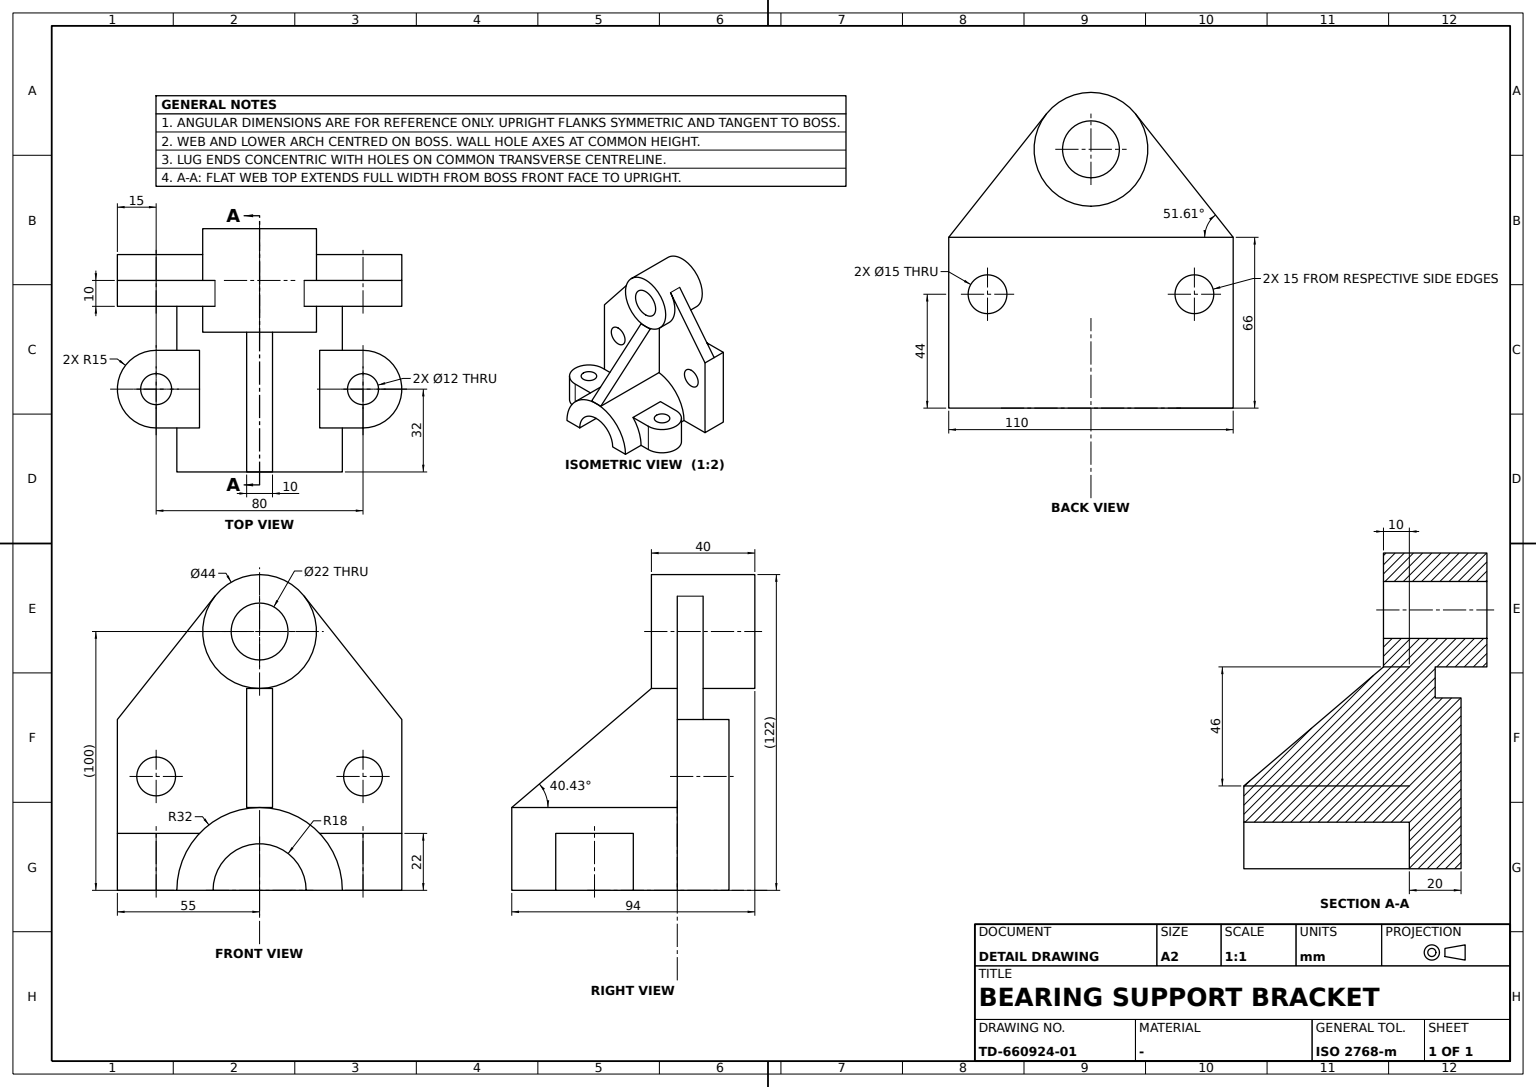
ISO-10303-21;
HEADER;
FILE_DESCRIPTION((''),'2;1');
FILE_NAME('','',(''),(''),'','','');
FILE_SCHEMA(('AUTOMOTIVE_DESIGN'));
ENDSEC;
DATA;
#1=APPLICATION_CONTEXT('');
#2=PRODUCT_CONTEXT('',#1,'mechanical');
#3=PRODUCT('','','',(#2));
#4=PRODUCT_DEFINITION_FORMATION('','',#3);
#5=PRODUCT_DEFINITION_CONTEXT('',#1,'design');
#6=PRODUCT_DEFINITION('','',#4,#5);
#7=PRODUCT_DEFINITION_SHAPE('','',#6);
#8=(LENGTH_UNIT()NAMED_UNIT(*)SI_UNIT(.MILLI.,.METRE.));
#9=(NAMED_UNIT(*)PLANE_ANGLE_UNIT()SI_UNIT($,.RADIAN.));
#10=(NAMED_UNIT(*)SI_UNIT($,.STERADIAN.)SOLID_ANGLE_UNIT());
#11=UNCERTAINTY_MEASURE_WITH_UNIT(LENGTH_MEASURE(0.005),#8,'distance_accuracy_value','');
#12=(GEOMETRIC_REPRESENTATION_CONTEXT(3)GLOBAL_UNCERTAINTY_ASSIGNED_CONTEXT((#11))GLOBAL_UNIT_ASSIGNED_CONTEXT((#8,#9,#10))REPRESENTATION_CONTEXT('',''));
#13=CARTESIAN_POINT('',(17.244825,-42.,113.660747));
#14=VERTEX_POINT('',#13);
#15=CARTESIAN_POINT('',(17.244825,-32.,113.660747));
#16=VERTEX_POINT('',#15);
#17=DIRECTION('',(0.,-1.,0.));
#18=VECTOR('',#17,1000.);
#19=LINE('',#13,#18);
#20=EDGE_CURVE('',#14,#16,#19,.F.);
#21=ORIENTED_EDGE('',*,*,#20,.F.);
#22=CARTESIAN_POINT('',(55.,-42.,66.));
#23=VERTEX_POINT('',#22);
#24=DIRECTION('',(0.620943034,0.,-0.783855694));
#25=VECTOR('',#24,1000.);
#26=LINE('',#13,#25);
#27=EDGE_CURVE('',#14,#23,#26,.T.);
#28=ORIENTED_EDGE('',*,*,#27,.T.);
#29=CARTESIAN_POINT('',(55.,-32.,66.));
#30=VERTEX_POINT('',#29);
#31=LINE('',#29,#18);
#32=EDGE_CURVE('',#30,#23,#31,.T.);
#33=ORIENTED_EDGE('',*,*,#32,.F.);
#34=LINE('',#15,#25);
#35=EDGE_CURVE('',#16,#30,#34,.T.);
#36=ORIENTED_EDGE('',*,*,#35,.F.);
#37=EDGE_LOOP('',(#21,#28,#33,#36));
#38=FACE_BOUND('',#37,.T.);
#39=DIRECTION('',(-0.783855694,0.,-0.620943034));
#40=AXIS2_PLACEMENT_3D('',#15,#39,#24);
#41=PLANE('',#40);
#42=ADVANCED_FACE('',(#38),#41,.F.);
#43=CARTESIAN_POINT('',(32.,32.,0.));
#44=VERTEX_POINT('',#43);
#45=CARTESIAN_POINT('',(18.,32.,0.));
#46=VERTEX_POINT('',#45);
#47=CARTESIAN_POINT('',(0.,32.,0.));
#48=DIRECTION('',(-1.,0.,0.));
#49=VECTOR('',#48,1000.);
#50=LINE('',#47,#49);
#51=EDGE_CURVE('',#44,#46,#50,.T.);
#52=ORIENTED_EDGE('',*,*,#51,.T.);
#53=CARTESIAN_POINT('',(-18.,32.,0.));
#54=VERTEX_POINT('',#53);
#55=DIRECTION('',(0.,1.,0.));
#56=DIRECTION('',(0.,0.,1.));
#57=AXIS2_PLACEMENT_3D('',#47,#55,#56);
#58=CIRCLE('',#57,18.);
#59=EDGE_CURVE('',#54,#46,#58,.T.);
#60=ORIENTED_EDGE('',*,*,#59,.F.);
#61=CARTESIAN_POINT('',(-32.,32.,0.));
#62=VERTEX_POINT('',#61);
#63=EDGE_CURVE('',#54,#62,#50,.T.);
#64=ORIENTED_EDGE('',*,*,#63,.T.);
#65=CIRCLE('',#57,32.);
#66=EDGE_CURVE('',#62,#44,#65,.T.);
#67=ORIENTED_EDGE('',*,*,#66,.T.);
#68=EDGE_LOOP('',(#52,#60,#64,#67));
#69=FACE_BOUND('',#68,.T.);
#70=AXIS2_PLACEMENT_3D('',#47,#55,#48);
#71=PLANE('',#70);
#72=ADVANCED_FACE('',(#69),#71,.T.);
#73=CARTESIAN_POINT('',(-32.,-15.,0.));
#74=VERTEX_POINT('',#73);
#75=CARTESIAN_POINT('',(-23.2379,-15.,22.));
#76=VERTEX_POINT('',#75);
#77=CARTESIAN_POINT('',(0.,-15.,0.));
#78=AXIS2_PLACEMENT_3D('',#77,#55,#56);
#79=CIRCLE('',#78,32.);
#80=EDGE_CURVE('',#74,#76,#79,.T.);
#81=ORIENTED_EDGE('',*,*,#80,.F.);
#82=CARTESIAN_POINT('',(-32.,-32.,0.));
#83=VERTEX_POINT('',#82);
#84=VECTOR('',#55,1000.);
#85=LINE('',#82,#84);
#86=EDGE_CURVE('',#74,#83,#85,.F.);
#87=ORIENTED_EDGE('',*,*,#86,.T.);
#88=CARTESIAN_POINT('',(0.,-32.,32.));
#89=VERTEX_POINT('',#88);
#90=CARTESIAN_POINT('',(0.,-32.,0.));
#91=AXIS2_PLACEMENT_3D('',#90,#55,#56);
#92=CIRCLE('',#91,32.);
#93=EDGE_CURVE('',#83,#89,#92,.T.);
#94=ORIENTED_EDGE('',*,*,#93,.T.);
#95=CARTESIAN_POINT('',(32.,-32.,0.));
#96=VERTEX_POINT('',#95);
#97=EDGE_CURVE('',#89,#96,#92,.T.);
#98=ORIENTED_EDGE('',*,*,#97,.T.);
#99=CARTESIAN_POINT('',(32.,-15.,0.));
#100=VERTEX_POINT('',#99);
#101=LINE('',#95,#84);
#102=EDGE_CURVE('',#96,#100,#101,.T.);
#103=ORIENTED_EDGE('',*,*,#102,.T.);
#104=CARTESIAN_POINT('',(23.2379,-15.,22.));
#105=VERTEX_POINT('',#104);
#106=EDGE_CURVE('',#105,#100,#79,.T.);
#107=ORIENTED_EDGE('',*,*,#106,.F.);
#108=CARTESIAN_POINT('',(23.2379,15.,22.));
#109=VERTEX_POINT('',#108);
#110=LINE('',#104,#84);
#111=EDGE_CURVE('',#105,#109,#110,.T.);
#112=ORIENTED_EDGE('',*,*,#111,.T.);
#113=CARTESIAN_POINT('',(32.,15.,0.));
#114=VERTEX_POINT('',#113);
#115=CARTESIAN_POINT('',(0.,15.,0.));
#116=DIRECTION('',(1.,0.,0.));
#117=AXIS2_PLACEMENT_3D('',#115,#17,#116);
#118=CIRCLE('',#117,32.);
#119=EDGE_CURVE('',#114,#109,#118,.T.);
#120=ORIENTED_EDGE('',*,*,#119,.F.);
#121=LINE('',#113,#84);
#122=EDGE_CURVE('',#114,#44,#121,.T.);
#123=ORIENTED_EDGE('',*,*,#122,.T.);
#124=ORIENTED_EDGE('',*,*,#66,.F.);
#125=CARTESIAN_POINT('',(-32.,15.,0.));
#126=VERTEX_POINT('',#125);
#127=LINE('',#125,#84);
#128=EDGE_CURVE('',#62,#126,#127,.F.);
#129=ORIENTED_EDGE('',*,*,#128,.T.);
#130=CARTESIAN_POINT('',(-23.2379,15.,22.));
#131=VERTEX_POINT('',#130);
#132=EDGE_CURVE('',#131,#126,#118,.T.);
#133=ORIENTED_EDGE('',*,*,#132,.F.);
#134=LINE('',#75,#84);
#135=EDGE_CURVE('',#76,#131,#134,.T.);
#136=ORIENTED_EDGE('',*,*,#135,.F.);
#137=EDGE_LOOP('',(#81,#87,#94,#98,#103,#107,#112,#120,#123,#124,#129,#133,#136));
#138=FACE_BOUND('',#137,.T.);
#139=CARTESIAN_POINT('',(0.,0.,0.));
#140=AXIS2_PLACEMENT_3D('',#139,#55,#48);
#141=CYLINDRICAL_SURFACE('',#140,32.);
#142=ADVANCED_FACE('',(#138),#141,.T.);
#143=ORIENTED_EDGE('',*,*,#93,.F.);
#144=CARTESIAN_POINT('',(-55.,-32.,0.));
#145=VERTEX_POINT('',#144);
#146=VECTOR('',#116,1000.);
#147=LINE('',#95,#146);
#148=EDGE_CURVE('',#145,#83,#147,.T.);
#149=ORIENTED_EDGE('',*,*,#148,.F.);
#150=CARTESIAN_POINT('',(-55.,-32.,66.));
#151=VERTEX_POINT('',#150);
#152=DIRECTION('',(0.,0.,-1.));
#153=VECTOR('',#152,1000.);
#154=LINE('',#150,#153);
#155=EDGE_CURVE('',#151,#145,#154,.T.);
#156=ORIENTED_EDGE('',*,*,#155,.F.);
#157=CARTESIAN_POINT('',(-17.244825,-32.,113.660747));
#158=VERTEX_POINT('',#157);
#159=DIRECTION('',(0.620943034,0.,0.783855694));
#160=VECTOR('',#159,1000.);
#161=LINE('',#150,#160);
#162=EDGE_CURVE('',#151,#158,#161,.T.);
#163=ORIENTED_EDGE('',*,*,#162,.T.);
#164=CARTESIAN_POINT('',(0.,-32.,78.));
#165=VERTEX_POINT('',#164);
#166=CARTESIAN_POINT('',(0.,-32.,100.));
#167=AXIS2_PLACEMENT_3D('',#166,#55,#56);
#168=CIRCLE('',#167,22.);
#169=EDGE_CURVE('',#165,#158,#168,.T.);
#170=ORIENTED_EDGE('',*,*,#169,.F.);
#171=CARTESIAN_POINT('',(-5.,-32.,78.));
#172=VERTEX_POINT('',#171);
#173=LINE('',#164,#146);
#174=EDGE_CURVE('',#172,#165,#173,.T.);
#175=ORIENTED_EDGE('',*,*,#174,.F.);
#176=CARTESIAN_POINT('',(-5.,-32.,32.));
#177=VERTEX_POINT('',#176);
#178=CARTESIAN_POINT('',(-5.,-32.,0.));
#179=LINE('',#178,#153);
#180=EDGE_CURVE('',#172,#177,#179,.T.);
#181=ORIENTED_EDGE('',*,*,#180,.T.);
#182=LINE('',#88,#146);
#183=EDGE_CURVE('',#177,#89,#182,.T.);
#184=ORIENTED_EDGE('',*,*,#183,.T.);
#185=EDGE_LOOP('',(#143,#149,#156,#163,#170,#175,#181,#184));
#186=FACE_BOUND('',#185,.T.);
#187=CARTESIAN_POINT('',(-40.,-32.,51.5));
#188=VERTEX_POINT('',#187);
#189=CARTESIAN_POINT('',(-40.,-32.,44.));
#190=AXIS2_PLACEMENT_3D('',#189,#55,#56);
#191=CIRCLE('',#190,7.5);
#192=EDGE_CURVE('',#188,#188,#191,.T.);
#193=ORIENTED_EDGE('',*,*,#192,.F.);
#194=EDGE_LOOP('',(#193));
#195=FACE_BOUND('',#194,.T.);
#196=AXIS2_PLACEMENT_3D('',#90,#55,#48);
#197=PLANE('',#196);
#198=ADVANCED_FACE('',(#186,#195),#197,.T.);
#199=CARTESIAN_POINT('',(5.,-32.,78.));
#200=VERTEX_POINT('',#199);
#201=EDGE_CURVE('',#165,#200,#173,.T.);
#202=ORIENTED_EDGE('',*,*,#201,.T.);
#203=CARTESIAN_POINT('',(5.,-22.,78.));
#204=VERTEX_POINT('',#203);
#205=CARTESIAN_POINT('',(5.,0.,78.));
#206=LINE('',#205,#18);
#207=EDGE_CURVE('',#204,#200,#206,.T.);
#208=ORIENTED_EDGE('',*,*,#207,.F.);
#209=CARTESIAN_POINT('',(-5.,-22.,78.));
#210=VERTEX_POINT('',#209);
#211=CARTESIAN_POINT('',(0.,-22.,78.));
#212=LINE('',#211,#146);
#213=EDGE_CURVE('',#210,#204,#212,.T.);
#214=ORIENTED_EDGE('',*,*,#213,.F.);
#215=CARTESIAN_POINT('',(-5.,0.,78.));
#216=LINE('',#215,#18);
#217=EDGE_CURVE('',#210,#172,#216,.T.);
#218=ORIENTED_EDGE('',*,*,#217,.T.);
#219=ORIENTED_EDGE('',*,*,#174,.T.);
#220=EDGE_LOOP('',(#202,#208,#214,#218,#219));
#221=FACE_BOUND('',#220,.T.);
#222=AXIS2_PLACEMENT_3D('',#211,#56,#17);
#223=PLANE('',#222);
#224=ADVANCED_FACE('',(#221),#223,.T.);
#225=CARTESIAN_POINT('',(-34.,0.,22.));
#226=VERTEX_POINT('',#225);
#227=CARTESIAN_POINT('',(-40.,0.,22.));
#228=AXIS2_PLACEMENT_3D('',#227,#56,#116);
#229=CIRCLE('',#228,6.);
#230=EDGE_CURVE('',#226,#226,#229,.F.);
#231=ORIENTED_EDGE('',*,*,#230,.T.);
#232=EDGE_LOOP('',(#231));
#233=FACE_BOUND('',#232,.T.);
#234=CARTESIAN_POINT('',(-40.,-15.,22.));
#235=VERTEX_POINT('',#234);
#236=CARTESIAN_POINT('',(-40.,15.,22.));
#237=VERTEX_POINT('',#236);
#238=CIRCLE('',#228,15.);
#239=EDGE_CURVE('',#235,#237,#238,.F.);
#240=ORIENTED_EDGE('',*,*,#239,.F.);
#241=CARTESIAN_POINT('',(40.,-15.,22.));
#242=LINE('',#241,#146);
#243=EDGE_CURVE('',#235,#76,#242,.T.);
#244=ORIENTED_EDGE('',*,*,#243,.T.);
#245=ORIENTED_EDGE('',*,*,#135,.T.);
#246=CARTESIAN_POINT('',(20.,15.,22.));
#247=LINE('',#246,#49);
#248=EDGE_CURVE('',#131,#237,#247,.T.);
#249=ORIENTED_EDGE('',*,*,#248,.T.);
#250=EDGE_LOOP('',(#240,#244,#245,#249));
#251=FACE_BOUND('',#250,.T.);
#252=CARTESIAN_POINT('',(0.,0.,22.));
#253=AXIS2_PLACEMENT_3D('',#252,#56,#55);
#254=PLANE('',#253);
#255=ADVANCED_FACE('',(#233,#251),#254,.T.);
#256=ORIENTED_EDGE('',*,*,#119,.T.);
#257=CARTESIAN_POINT('',(40.,15.,22.));
#258=VERTEX_POINT('',#257);
#259=CARTESIAN_POINT('',(0.,15.,22.));
#260=LINE('',#259,#146);
#261=EDGE_CURVE('',#109,#258,#260,.T.);
#262=ORIENTED_EDGE('',*,*,#261,.T.);
#263=CARTESIAN_POINT('',(40.,15.,0.));
#264=VERTEX_POINT('',#263);
#265=CARTESIAN_POINT('',(40.,15.,11.));
#266=VECTOR('',#56,1000.);
#267=LINE('',#265,#266);
#268=EDGE_CURVE('',#264,#258,#267,.T.);
#269=ORIENTED_EDGE('',*,*,#268,.F.);
#270=CARTESIAN_POINT('',(20.,15.,0.));
#271=LINE('',#270,#146);
#272=EDGE_CURVE('',#114,#264,#271,.T.);
#273=ORIENTED_EDGE('',*,*,#272,.F.);
#274=EDGE_LOOP('',(#256,#262,#269,#273));
#275=FACE_BOUND('',#274,.T.);
#276=AXIS2_PLACEMENT_3D('',#270,#17,#116);
#277=PLANE('',#276);
#278=ADVANCED_FACE('',(#275),#277,.F.);
#279=ORIENTED_EDGE('',*,*,#162,.F.);
#280=CARTESIAN_POINT('',(-55.,-42.,66.));
#281=VERTEX_POINT('',#280);
#282=LINE('',#150,#18);
#283=EDGE_CURVE('',#151,#281,#282,.T.);
#284=ORIENTED_EDGE('',*,*,#283,.T.);
#285=CARTESIAN_POINT('',(-17.244825,-42.,113.660747));
#286=VERTEX_POINT('',#285);
#287=LINE('',#280,#160);
#288=EDGE_CURVE('',#281,#286,#287,.T.);
#289=ORIENTED_EDGE('',*,*,#288,.T.);
#290=LINE('',#285,#18);
#291=EDGE_CURVE('',#286,#158,#290,.F.);
#292=ORIENTED_EDGE('',*,*,#291,.T.);
#293=EDGE_LOOP('',(#279,#284,#289,#292));
#294=FACE_BOUND('',#293,.T.);
#295=DIRECTION('',(0.783855694,0.,-0.620943034));
#296=AXIS2_PLACEMENT_3D('',#150,#295,#159);
#297=PLANE('',#296);
#298=ADVANCED_FACE('',(#294),#297,.F.);
#299=CARTESIAN_POINT('',(-5.,32.,32.));
#300=VERTEX_POINT('',#299);
#301=CARTESIAN_POINT('',(5.,32.,32.));
#302=VERTEX_POINT('',#301);
#303=CARTESIAN_POINT('',(0.,32.,32.));
#304=LINE('',#303,#146);
#305=EDGE_CURVE('',#300,#302,#304,.T.);
#306=ORIENTED_EDGE('',*,*,#305,.T.);
#307=CARTESIAN_POINT('',(5.,-32.,32.));
#308=VERTEX_POINT('',#307);
#309=CARTESIAN_POINT('',(5.,0.,32.));
#310=LINE('',#309,#84);
#311=EDGE_CURVE('',#308,#302,#310,.T.);
#312=ORIENTED_EDGE('',*,*,#311,.F.);
#313=EDGE_CURVE('',#89,#308,#182,.T.);
#314=ORIENTED_EDGE('',*,*,#313,.F.);
#315=ORIENTED_EDGE('',*,*,#183,.F.);
#316=CARTESIAN_POINT('',(-5.,0.,32.));
#317=LINE('',#316,#84);
#318=EDGE_CURVE('',#177,#300,#317,.T.);
#319=ORIENTED_EDGE('',*,*,#318,.T.);
#320=EDGE_LOOP('',(#306,#312,#314,#315,#319));
#321=FACE_BOUND('',#320,.T.);
#322=AXIS2_PLACEMENT_3D('',#88,#152,#55);
#323=PLANE('',#322);
#324=ADVANCED_FACE('',(#321),#323,.T.);
#325=CARTESIAN_POINT('',(-18.,-32.,0.));
#326=VERTEX_POINT('',#325);
#327=CARTESIAN_POINT('',(18.,-32.,0.));
#328=VERTEX_POINT('',#327);
#329=EDGE_CURVE('',#326,#328,#147,.T.);
#330=ORIENTED_EDGE('',*,*,#329,.F.);
#331=CIRCLE('',#91,18.);
#332=EDGE_CURVE('',#326,#328,#331,.T.);
#333=ORIENTED_EDGE('',*,*,#332,.T.);
#334=EDGE_LOOP('',(#330,#333));
#335=FACE_BOUND('',#334,.T.);
#336=ADVANCED_FACE('',(#335),#197,.T.);
#337=CARTESIAN_POINT('',(-40.,15.,0.));
#338=VERTEX_POINT('',#337);
#339=LINE('',#113,#49);
#340=EDGE_CURVE('',#126,#338,#339,.T.);
#341=ORIENTED_EDGE('',*,*,#340,.T.);
#342=CARTESIAN_POINT('',(-40.,15.,11.));
#343=LINE('',#342,#153);
#344=EDGE_CURVE('',#338,#237,#343,.F.);
#345=ORIENTED_EDGE('',*,*,#344,.T.);
#346=ORIENTED_EDGE('',*,*,#248,.F.);
#347=ORIENTED_EDGE('',*,*,#132,.T.);
#348=EDGE_LOOP('',(#341,#345,#346,#347));
#349=FACE_BOUND('',#348,.T.);
#350=ADVANCED_FACE('',(#349),#277,.F.);
#351=CARTESIAN_POINT('',(-55.,-52.,66.));
#352=VERTEX_POINT('',#351);
#353=EDGE_CURVE('',#281,#352,#282,.T.);
#354=ORIENTED_EDGE('',*,*,#353,.F.);
#355=ORIENTED_EDGE('',*,*,#283,.F.);
#356=ORIENTED_EDGE('',*,*,#155,.T.);
#357=CARTESIAN_POINT('',(-55.,-52.,0.));
#358=VERTEX_POINT('',#357);
#359=LINE('',#144,#18);
#360=EDGE_CURVE('',#145,#358,#359,.T.);
#361=ORIENTED_EDGE('',*,*,#360,.T.);
#362=LINE('',#357,#153);
#363=EDGE_CURVE('',#352,#358,#362,.T.);
#364=ORIENTED_EDGE('',*,*,#363,.F.);
#365=EDGE_LOOP('',(#354,#355,#356,#361,#364));
#366=FACE_BOUND('',#365,.T.);
#367=AXIS2_PLACEMENT_3D('',#150,#48,#152);
#368=PLANE('',#367);
#369=ADVANCED_FACE('',(#366),#368,.T.);
#370=ORIENTED_EDGE('',*,*,#111,.F.);
#371=VERTEX_POINT('',#241);
#372=CARTESIAN_POINT('',(0.,-15.,22.));
#373=LINE('',#372,#49);
#374=EDGE_CURVE('',#371,#105,#373,.T.);
#375=ORIENTED_EDGE('',*,*,#374,.F.);
#376=CARTESIAN_POINT('',(40.,0.,22.));
#377=AXIS2_PLACEMENT_3D('',#376,#56,#116);
#378=CIRCLE('',#377,15.);
#379=EDGE_CURVE('',#371,#258,#378,.T.);
#380=ORIENTED_EDGE('',*,*,#379,.T.);
#381=ORIENTED_EDGE('',*,*,#261,.F.);
#382=EDGE_LOOP('',(#370,#375,#380,#381));
#383=FACE_BOUND('',#382,.T.);
#384=CARTESIAN_POINT('',(46.,0.,22.));
#385=VERTEX_POINT('',#384);
#386=CIRCLE('',#377,6.);
#387=EDGE_CURVE('',#385,#385,#386,.T.);
#388=ORIENTED_EDGE('',*,*,#387,.F.);
#389=EDGE_LOOP('',(#388));
#390=FACE_BOUND('',#389,.T.);
#391=ADVANCED_FACE('',(#383,#390),#254,.T.);
#392=CARTESIAN_POINT('',(40.,-15.,0.));
#393=VERTEX_POINT('',#392);
#394=LINE('',#392,#49);
#395=EDGE_CURVE('',#393,#100,#394,.T.);
#396=ORIENTED_EDGE('',*,*,#395,.F.);
#397=CARTESIAN_POINT('',(40.,-15.,11.));
#398=LINE('',#397,#266);
#399=EDGE_CURVE('',#393,#371,#398,.T.);
#400=ORIENTED_EDGE('',*,*,#399,.T.);
#401=ORIENTED_EDGE('',*,*,#374,.T.);
#402=ORIENTED_EDGE('',*,*,#106,.T.);
#403=EDGE_LOOP('',(#396,#400,#401,#402));
#404=FACE_BOUND('',#403,.T.);
#405=AXIS2_PLACEMENT_3D('',#392,#55,#48);
#406=PLANE('',#405);
#407=ADVANCED_FACE('',(#404),#406,.F.);
#408=CARTESIAN_POINT('',(55.,-52.,0.));
#409=VERTEX_POINT('',#408);
#410=CARTESIAN_POINT('',(0.,-52.,0.));
#411=LINE('',#410,#146);
#412=EDGE_CURVE('',#358,#409,#411,.T.);
#413=ORIENTED_EDGE('',*,*,#412,.T.);
#414=CARTESIAN_POINT('',(55.,-52.,66.));
#415=VERTEX_POINT('',#414);
#416=LINE('',#408,#266);
#417=EDGE_CURVE('',#409,#415,#416,.T.);
#418=ORIENTED_EDGE('',*,*,#417,.T.);
#419=CARTESIAN_POINT('',(0.,-52.,66.));
#420=LINE('',#419,#49);
#421=EDGE_CURVE('',#415,#352,#420,.T.);
#422=ORIENTED_EDGE('',*,*,#421,.T.);
#423=ORIENTED_EDGE('',*,*,#363,.T.);
#424=EDGE_LOOP('',(#413,#418,#422,#423));
#425=FACE_BOUND('',#424,.T.);
#426=CARTESIAN_POINT('',(40.,-52.,36.5));
#427=VERTEX_POINT('',#426);
#428=CARTESIAN_POINT('',(40.,-52.,44.));
#429=AXIS2_PLACEMENT_3D('',#428,#17,#152);
#430=CIRCLE('',#429,7.5);
#431=EDGE_CURVE('',#427,#427,#430,.T.);
#432=ORIENTED_EDGE('',*,*,#431,.F.);
#433=EDGE_LOOP('',(#432));
#434=FACE_BOUND('',#433,.T.);
#435=CARTESIAN_POINT('',(-40.,-52.,36.5));
#436=VERTEX_POINT('',#435);
#437=CARTESIAN_POINT('',(-40.,-52.,44.));
#438=AXIS2_PLACEMENT_3D('',#437,#17,#152);
#439=CIRCLE('',#438,7.5);
#440=EDGE_CURVE('',#436,#436,#439,.T.);
#441=ORIENTED_EDGE('',*,*,#440,.F.);
#442=EDGE_LOOP('',(#441));
#443=FACE_BOUND('',#442,.T.);
#444=AXIS2_PLACEMENT_3D('',#410,#17,#116);
#445=PLANE('',#444);
#446=ADVANCED_FACE('',(#425,#434,#443),#445,.T.);
#447=CARTESIAN_POINT('',(0.,-42.,100.));
#448=AXIS2_PLACEMENT_3D('',#447,#55,#56);
#449=CIRCLE('',#448,22.);
#450=EDGE_CURVE('',#14,#286,#449,.T.);
#451=ORIENTED_EDGE('',*,*,#450,.T.);
#452=ORIENTED_EDGE('',*,*,#288,.F.);
#453=LINE('',#22,#49);
#454=EDGE_CURVE('',#23,#281,#453,.T.);
#455=ORIENTED_EDGE('',*,*,#454,.F.);
#456=ORIENTED_EDGE('',*,*,#27,.F.);
#457=EDGE_LOOP('',(#451,#452,#455,#456));
#458=FACE_BOUND('',#457,.T.);
#459=CARTESIAN_POINT('',(0.,-42.,0.));
#460=AXIS2_PLACEMENT_3D('',#459,#55,#48);
#461=PLANE('',#460);
#462=ADVANCED_FACE('',(#458),#461,.F.);
#463=CARTESIAN_POINT('',(-46.,0.,0.));
#464=VERTEX_POINT('',#463);
#465=CARTESIAN_POINT('',(-40.,0.,0.));
#466=AXIS2_PLACEMENT_3D('',#465,#152,#48);
#467=CIRCLE('',#466,6.);
#468=EDGE_CURVE('',#464,#464,#467,.T.);
#469=ORIENTED_EDGE('',*,*,#468,.T.);
#470=EDGE_LOOP('',(#469));
#471=FACE_BOUND('',#470,.T.);
#472=ORIENTED_EDGE('',*,*,#230,.F.);
#473=EDGE_LOOP('',(#472));
#474=FACE_BOUND('',#473,.T.);
#475=CARTESIAN_POINT('',(-40.,0.,11.));
#476=AXIS2_PLACEMENT_3D('',#475,#152,#55);
#477=CYLINDRICAL_SURFACE('',#476,6.);
#478=ADVANCED_FACE('',(#471,#474),#477,.F.);
#479=ORIENTED_EDGE('',*,*,#399,.F.);
#480=CARTESIAN_POINT('',(40.,0.,0.));
#481=AXIS2_PLACEMENT_3D('',#480,#152,#48);
#482=CIRCLE('',#481,15.);
#483=EDGE_CURVE('',#393,#264,#482,.F.);
#484=ORIENTED_EDGE('',*,*,#483,.T.);
#485=ORIENTED_EDGE('',*,*,#268,.T.);
#486=ORIENTED_EDGE('',*,*,#379,.F.);
#487=EDGE_LOOP('',(#479,#484,#485,#486));
#488=FACE_BOUND('',#487,.T.);
#489=CARTESIAN_POINT('',(40.,0.,11.));
#490=AXIS2_PLACEMENT_3D('',#489,#56,#55);
#491=CYLINDRICAL_SURFACE('',#490,15.);
#492=ADVANCED_FACE('',(#488),#491,.T.);
#493=ORIENTED_EDGE('',*,*,#32,.T.);
#494=EDGE_CURVE('',#23,#415,#31,.T.);
#495=ORIENTED_EDGE('',*,*,#494,.T.);
#496=ORIENTED_EDGE('',*,*,#417,.F.);
#497=CARTESIAN_POINT('',(55.,-32.,0.));
#498=VERTEX_POINT('',#497);
#499=CARTESIAN_POINT('',(55.,0.,0.));
#500=LINE('',#499,#18);
#501=EDGE_CURVE('',#498,#409,#500,.T.);
#502=ORIENTED_EDGE('',*,*,#501,.F.);
#503=LINE('',#497,#266);
#504=EDGE_CURVE('',#498,#30,#503,.T.);
#505=ORIENTED_EDGE('',*,*,#504,.T.);
#506=EDGE_LOOP('',(#493,#495,#496,#502,#505));
#507=FACE_BOUND('',#506,.T.);
#508=AXIS2_PLACEMENT_3D('',#497,#116,#56);
#509=PLANE('',#508);
#510=ADVANCED_FACE('',(#507),#509,.T.);
#511=CARTESIAN_POINT('',(40.,-32.,51.5));
#512=VERTEX_POINT('',#511);
#513=CARTESIAN_POINT('',(40.,-32.,44.));
#514=AXIS2_PLACEMENT_3D('',#513,#55,#56);
#515=CIRCLE('',#514,7.5);
#516=EDGE_CURVE('',#512,#512,#515,.T.);
#517=ORIENTED_EDGE('',*,*,#516,.F.);
#518=EDGE_LOOP('',(#517));
#519=FACE_BOUND('',#518,.T.);
#520=EDGE_CURVE('',#96,#498,#147,.T.);
#521=ORIENTED_EDGE('',*,*,#520,.F.);
#522=ORIENTED_EDGE('',*,*,#97,.F.);
#523=ORIENTED_EDGE('',*,*,#313,.T.);
#524=CARTESIAN_POINT('',(5.,-32.,0.));
#525=LINE('',#524,#153);
#526=EDGE_CURVE('',#200,#308,#525,.T.);
#527=ORIENTED_EDGE('',*,*,#526,.F.);
#528=ORIENTED_EDGE('',*,*,#201,.F.);
#529=EDGE_CURVE('',#16,#165,#168,.T.);
#530=ORIENTED_EDGE('',*,*,#529,.F.);
#531=ORIENTED_EDGE('',*,*,#35,.T.);
#532=ORIENTED_EDGE('',*,*,#504,.F.);
#533=EDGE_LOOP('',(#521,#522,#523,#527,#528,#530,#531,#532));
#534=FACE_BOUND('',#533,.T.);
#535=ADVANCED_FACE('',(#519,#534),#197,.T.);
#536=ORIENTED_EDGE('',*,*,#494,.F.);
#537=ORIENTED_EDGE('',*,*,#454,.T.);
#538=ORIENTED_EDGE('',*,*,#353,.T.);
#539=ORIENTED_EDGE('',*,*,#421,.F.);
#540=EDGE_LOOP('',(#536,#537,#538,#539));
#541=FACE_BOUND('',#540,.T.);
#542=AXIS2_PLACEMENT_3D('',#29,#56,#48);
#543=PLANE('',#542);
#544=ADVANCED_FACE('',(#541),#543,.T.);
#545=ORIENTED_EDGE('',*,*,#440,.T.);
#546=EDGE_LOOP('',(#545));
#547=FACE_BOUND('',#546,.T.);
#548=ORIENTED_EDGE('',*,*,#192,.T.);
#549=EDGE_LOOP('',(#548));
#550=FACE_BOUND('',#549,.T.);
#551=CARTESIAN_POINT('',(-40.,-32.1,44.));
#552=AXIS2_PLACEMENT_3D('',#551,#17,#116);
#553=CYLINDRICAL_SURFACE('',#552,7.5);
#554=ADVANCED_FACE('',(#547,#550),#553,.F.);
#555=CARTESIAN_POINT('',(0.,-22.,89.));
#556=VERTEX_POINT('',#555);
#557=CARTESIAN_POINT('',(0.,-22.,100.));
#558=AXIS2_PLACEMENT_3D('',#557,#17,#152);
#559=CIRCLE('',#558,11.);
#560=EDGE_CURVE('',#556,#556,#559,.T.);
#561=ORIENTED_EDGE('',*,*,#560,.F.);
#562=EDGE_LOOP('',(#561));
#563=FACE_BOUND('',#562,.T.);
#564=CARTESIAN_POINT('',(0.,-62.,89.));
#565=VERTEX_POINT('',#564);
#566=CARTESIAN_POINT('',(0.,-62.,100.));
#567=AXIS2_PLACEMENT_3D('',#566,#17,#152);
#568=CIRCLE('',#567,11.);
#569=EDGE_CURVE('',#565,#565,#568,.T.);
#570=ORIENTED_EDGE('',*,*,#569,.T.);
#571=EDGE_LOOP('',(#570));
#572=FACE_BOUND('',#571,.T.);
#573=AXIS2_PLACEMENT_3D('',#447,#17,#116);
#574=CYLINDRICAL_SURFACE('',#573,11.);
#575=ADVANCED_FACE('',(#563,#572),#574,.F.);
#576=ORIENTED_EDGE('',*,*,#318,.F.);
#577=ORIENTED_EDGE('',*,*,#180,.F.);
#578=ORIENTED_EDGE('',*,*,#217,.F.);
#579=CARTESIAN_POINT('',(-5.,29.252782,34.340223));
#580=DIRECTION('',(0.,0.76124323,-0.648466456));
#581=VECTOR('',#580,1000.);
#582=LINE('',#579,#581);
#583=EDGE_CURVE('',#210,#300,#582,.T.);
#584=ORIENTED_EDGE('',*,*,#583,.T.);
#585=EDGE_LOOP('',(#576,#577,#578,#584));
#586=FACE_BOUND('',#585,.T.);
#587=CARTESIAN_POINT('',(-5.,0.,0.));
#588=AXIS2_PLACEMENT_3D('',#587,#116,#55);
#589=PLANE('',#588);
#590=ADVANCED_FACE('',(#586),#589,.F.);
#591=ORIENTED_EDGE('',*,*,#516,.T.);
#592=EDGE_LOOP('',(#591));
#593=FACE_BOUND('',#592,.T.);
#594=ORIENTED_EDGE('',*,*,#431,.T.);
#595=EDGE_LOOP('',(#594));
#596=FACE_BOUND('',#595,.T.);
#597=CARTESIAN_POINT('',(40.,-32.1,44.));
#598=AXIS2_PLACEMENT_3D('',#597,#17,#116);
#599=CYLINDRICAL_SURFACE('',#598,7.5);
#600=ADVANCED_FACE('',(#593,#596),#599,.F.);
#601=ORIENTED_EDGE('',*,*,#583,.F.);
#602=ORIENTED_EDGE('',*,*,#213,.T.);
#603=CARTESIAN_POINT('',(5.,29.252782,34.340223));
#604=LINE('',#603,#581);
#605=EDGE_CURVE('',#204,#302,#604,.T.);
#606=ORIENTED_EDGE('',*,*,#605,.T.);
#607=ORIENTED_EDGE('',*,*,#305,.F.);
#608=EDGE_LOOP('',(#601,#602,#606,#607));
#609=FACE_BOUND('',#608,.T.);
#610=DIRECTION('',(0.,-0.648466456,-0.76124323));
#611=AXIS2_PLACEMENT_3D('',#211,#610,#580);
#612=PLANE('',#611);
#613=ADVANCED_FACE('',(#609),#612,.F.);
#614=ORIENTED_EDGE('',*,*,#569,.F.);
#615=EDGE_LOOP('',(#614));
#616=FACE_BOUND('',#615,.T.);
#617=CARTESIAN_POINT('',(0.,-62.,78.));
#618=VERTEX_POINT('',#617);
#619=CIRCLE('',#567,22.);
#620=EDGE_CURVE('',#618,#618,#619,.T.);
#621=ORIENTED_EDGE('',*,*,#620,.T.);
#622=EDGE_LOOP('',(#621));
#623=FACE_BOUND('',#622,.T.);
#624=CARTESIAN_POINT('',(0.,-62.,0.));
#625=AXIS2_PLACEMENT_3D('',#624,#17,#116);
#626=PLANE('',#625);
#627=ADVANCED_FACE('',(#616,#623),#626,.T.);
#628=VERTEX_POINT('',#211);
#629=CIRCLE('',#558,22.);
#630=EDGE_CURVE('',#628,#628,#629,.T.);
#631=ORIENTED_EDGE('',*,*,#630,.F.);
#632=EDGE_LOOP('',(#631));
#633=FACE_BOUND('',#632,.T.);
#634=ORIENTED_EDGE('',*,*,#560,.T.);
#635=EDGE_LOOP('',(#634));
#636=FACE_BOUND('',#635,.T.);
#637=CARTESIAN_POINT('',(0.,-22.,0.));
#638=AXIS2_PLACEMENT_3D('',#637,#17,#116);
#639=PLANE('',#638);
#640=ADVANCED_FACE('',(#633,#636),#639,.F.);
#641=ORIENTED_EDGE('',*,*,#387,.T.);
#642=EDGE_LOOP('',(#641));
#643=FACE_BOUND('',#642,.T.);
#644=CARTESIAN_POINT('',(34.,0.,0.));
#645=VERTEX_POINT('',#644);
#646=CIRCLE('',#481,6.);
#647=EDGE_CURVE('',#645,#645,#646,.F.);
#648=ORIENTED_EDGE('',*,*,#647,.F.);
#649=EDGE_LOOP('',(#648));
#650=FACE_BOUND('',#649,.T.);
#651=CYLINDRICAL_SURFACE('',#490,6.);
#652=ADVANCED_FACE('',(#643,#650),#651,.F.);
#653=ORIENTED_EDGE('',*,*,#243,.F.);
#654=CARTESIAN_POINT('',(-40.,-15.,0.));
#655=VERTEX_POINT('',#654);
#656=CARTESIAN_POINT('',(-40.,-15.,11.));
#657=LINE('',#656,#153);
#658=EDGE_CURVE('',#655,#235,#657,.F.);
#659=ORIENTED_EDGE('',*,*,#658,.F.);
#660=LINE('',#99,#146);
#661=EDGE_CURVE('',#655,#74,#660,.T.);
#662=ORIENTED_EDGE('',*,*,#661,.T.);
#663=ORIENTED_EDGE('',*,*,#80,.T.);
#664=EDGE_LOOP('',(#653,#659,#662,#663));
#665=FACE_BOUND('',#664,.T.);
#666=ADVANCED_FACE('',(#665),#406,.F.);
#667=ORIENTED_EDGE('',*,*,#658,.T.);
#668=ORIENTED_EDGE('',*,*,#239,.T.);
#669=ORIENTED_EDGE('',*,*,#344,.F.);
#670=CIRCLE('',#466,15.);
#671=EDGE_CURVE('',#655,#338,#670,.T.);
#672=ORIENTED_EDGE('',*,*,#671,.F.);
#673=EDGE_LOOP('',(#667,#668,#669,#672));
#674=FACE_BOUND('',#673,.T.);
#675=CYLINDRICAL_SURFACE('',#476,15.);
#676=ADVANCED_FACE('',(#674),#675,.T.);
#677=ORIENTED_EDGE('',*,*,#291,.F.);
#678=ORIENTED_EDGE('',*,*,#450,.F.);
#679=ORIENTED_EDGE('',*,*,#20,.T.);
#680=ORIENTED_EDGE('',*,*,#529,.T.);
#681=ORIENTED_EDGE('',*,*,#169,.T.);
#682=EDGE_LOOP('',(#677,#678,#679,#680,#681));
#683=FACE_BOUND('',#682,.T.);
#684=ORIENTED_EDGE('',*,*,#620,.F.);
#685=EDGE_LOOP('',(#684));
#686=FACE_BOUND('',#685,.T.);
#687=ORIENTED_EDGE('',*,*,#630,.T.);
#688=EDGE_LOOP('',(#687));
#689=FACE_BOUND('',#688,.T.);
#690=CYLINDRICAL_SURFACE('',#573,22.);
#691=ADVANCED_FACE('',(#683,#686,#689),#690,.T.);
#692=ORIENTED_EDGE('',*,*,#526,.T.);
#693=ORIENTED_EDGE('',*,*,#311,.T.);
#694=ORIENTED_EDGE('',*,*,#605,.F.);
#695=ORIENTED_EDGE('',*,*,#207,.T.);
#696=EDGE_LOOP('',(#692,#693,#694,#695));
#697=FACE_BOUND('',#696,.T.);
#698=CARTESIAN_POINT('',(5.,0.,0.));
#699=AXIS2_PLACEMENT_3D('',#698,#116,#55);
#700=PLANE('',#699);
#701=ADVANCED_FACE('',(#697),#700,.T.);
#702=LINE('',#325,#84);
#703=EDGE_CURVE('',#54,#326,#702,.F.);
#704=ORIENTED_EDGE('',*,*,#703,.F.);
#705=ORIENTED_EDGE('',*,*,#59,.T.);
#706=LINE('',#327,#84);
#707=EDGE_CURVE('',#328,#46,#706,.T.);
#708=ORIENTED_EDGE('',*,*,#707,.F.);
#709=ORIENTED_EDGE('',*,*,#332,.F.);
#710=EDGE_LOOP('',(#704,#705,#708,#709));
#711=FACE_BOUND('',#710,.T.);
#712=CYLINDRICAL_SURFACE('',#140,18.);
#713=ADVANCED_FACE('',(#711),#712,.F.);
#714=ORIENTED_EDGE('',*,*,#468,.F.);
#715=EDGE_LOOP('',(#714));
#716=FACE_BOUND('',#715,.T.);
#717=ORIENTED_EDGE('',*,*,#647,.T.);
#718=EDGE_LOOP('',(#717));
#719=FACE_BOUND('',#718,.T.);
#720=ORIENTED_EDGE('',*,*,#128,.F.);
#721=ORIENTED_EDGE('',*,*,#63,.F.);
#722=ORIENTED_EDGE('',*,*,#703,.T.);
#723=ORIENTED_EDGE('',*,*,#329,.T.);
#724=ORIENTED_EDGE('',*,*,#707,.T.);
#725=ORIENTED_EDGE('',*,*,#51,.F.);
#726=ORIENTED_EDGE('',*,*,#122,.F.);
#727=ORIENTED_EDGE('',*,*,#272,.T.);
#728=ORIENTED_EDGE('',*,*,#483,.F.);
#729=ORIENTED_EDGE('',*,*,#395,.T.);
#730=ORIENTED_EDGE('',*,*,#102,.F.);
#731=ORIENTED_EDGE('',*,*,#520,.T.);
#732=ORIENTED_EDGE('',*,*,#501,.T.);
#733=ORIENTED_EDGE('',*,*,#412,.F.);
#734=ORIENTED_EDGE('',*,*,#360,.F.);
#735=ORIENTED_EDGE('',*,*,#148,.T.);
#736=ORIENTED_EDGE('',*,*,#86,.F.);
#737=ORIENTED_EDGE('',*,*,#661,.F.);
#738=ORIENTED_EDGE('',*,*,#671,.T.);
#739=ORIENTED_EDGE('',*,*,#340,.F.);
#740=EDGE_LOOP('',(#720,#721,#722,#723,#724,#725,#726,#727,#728,#729,#730,#731,#732,#733,#734,#735,#736,#737,#738,#739));
#741=FACE_BOUND('',#740,.T.);
#742=CARTESIAN_POINT('',(32.,0.,0.));
#743=AXIS2_PLACEMENT_3D('',#742,#152,#48);
#744=PLANE('',#743);
#745=ADVANCED_FACE('',(#716,#719,#741),#744,.T.);
#746=CLOSED_SHELL('',(#42,#72,#142,#198,#224,#255,#278,#298,#324,#336,#350,#369,#391,#407,#446,#462,#478,#492,#510,#535,#544,#554,#575,#590,#600,#613,#627,#640,#652,#666,#676,#691,#701,#713,#745));
#747=MANIFOLD_SOLID_BREP('',#746);
#748=ADVANCED_BREP_SHAPE_REPRESENTATION('',(#747),#12);
#749=SHAPE_DEFINITION_REPRESENTATION(#7,#748);
ENDSEC;
END-ISO-10303-21;
